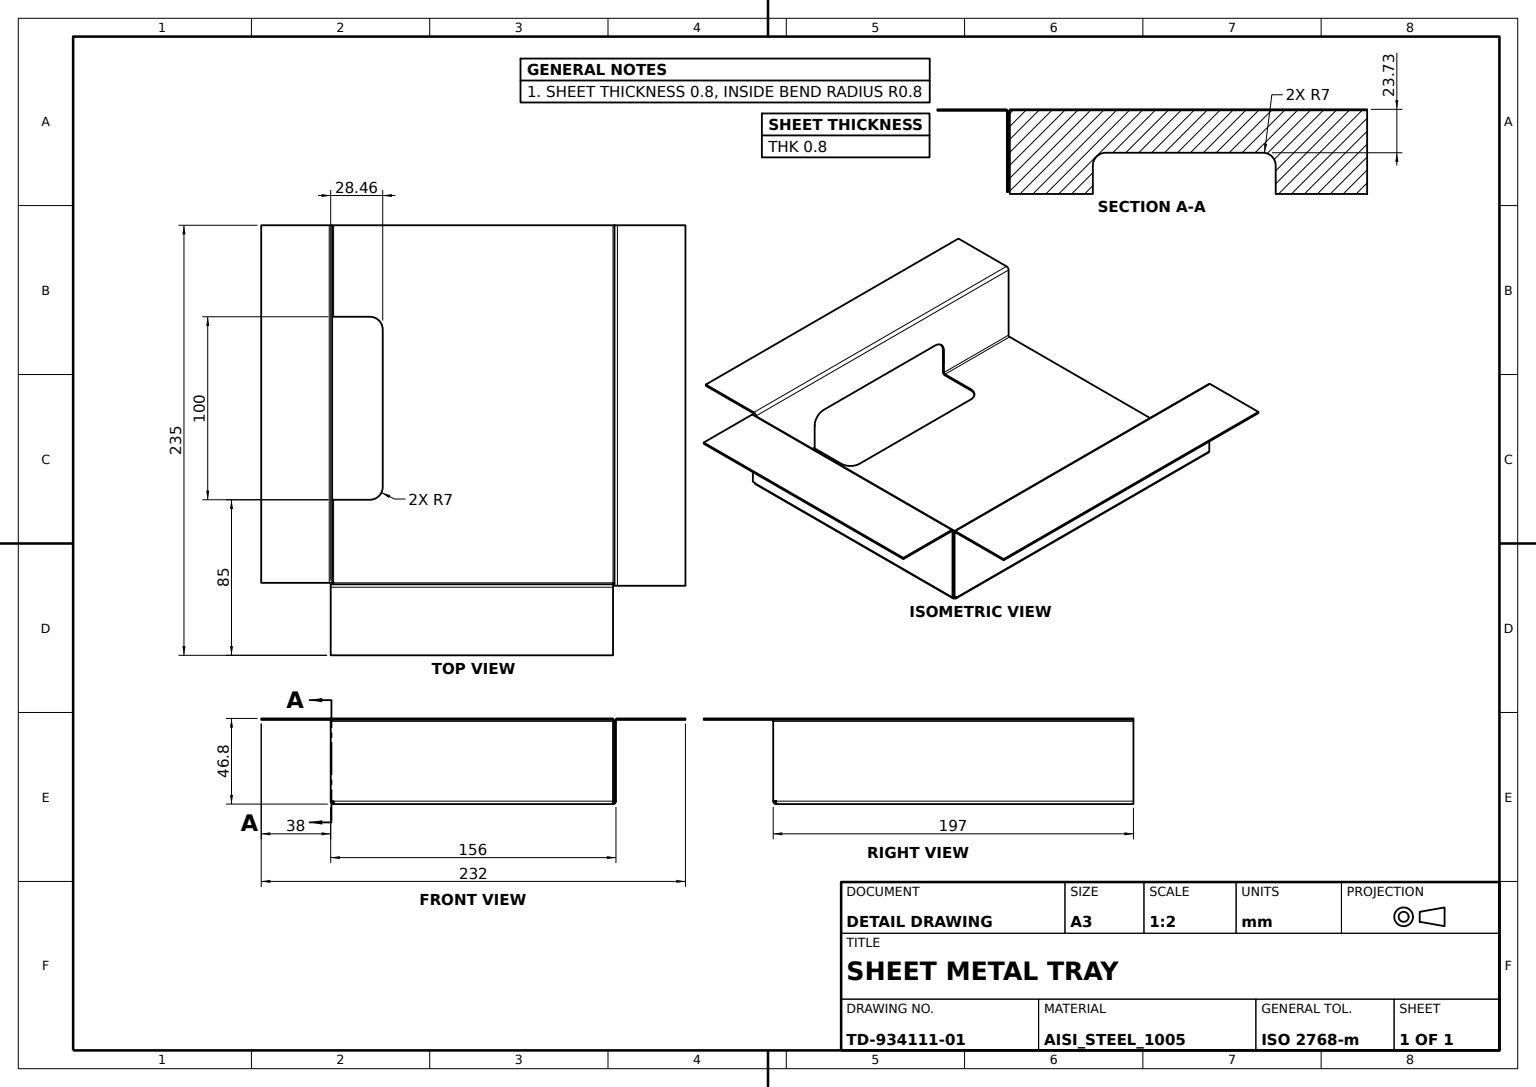
ISO-10303-21;
HEADER;
FILE_DESCRIPTION((''),'2;1');
FILE_NAME('','',(''),(''),'','','');
FILE_SCHEMA(('AUTOMOTIVE_DESIGN'));
ENDSEC;
DATA;
#1=APPLICATION_CONTEXT('');
#2=PRODUCT_CONTEXT('',#1,'mechanical');
#3=PRODUCT('','','',(#2));
#4=PRODUCT_DEFINITION_FORMATION('','',#3);
#5=PRODUCT_DEFINITION_CONTEXT('',#1,'design');
#6=PRODUCT_DEFINITION('','',#4,#5);
#7=PRODUCT_DEFINITION_SHAPE('','',#6);
#8=(LENGTH_UNIT()NAMED_UNIT(*)SI_UNIT(.MILLI.,.METRE.));
#9=(NAMED_UNIT(*)PLANE_ANGLE_UNIT()SI_UNIT($,.RADIAN.));
#10=(NAMED_UNIT(*)SI_UNIT($,.STERADIAN.)SOLID_ANGLE_UNIT());
#11=UNCERTAINTY_MEASURE_WITH_UNIT(LENGTH_MEASURE(0.005),#8,'distance_accuracy_value','');
#12=(GEOMETRIC_REPRESENTATION_CONTEXT(3)GLOBAL_UNCERTAINTY_ASSIGNED_CONTEXT((#11))GLOBAL_UNIT_ASSIGNED_CONTEXT((#8,#9,#10))REPRESENTATION_CONTEXT('',''));
#13=CARTESIAN_POINT('',(77.2,-98.5,1.6));
#14=VERTEX_POINT('',#13);
#15=CARTESIAN_POINT('',(77.2,-98.5,45.2));
#16=VERTEX_POINT('',#15);
#17=DIRECTION('',(0.,0.,1.));
#18=VECTOR('',#17,1000.);
#19=LINE('',#13,#18);
#20=EDGE_CURVE('',#14,#16,#19,.T.);
#21=ORIENTED_EDGE('',*,*,#20,.T.);
#22=CARTESIAN_POINT('',(77.2,98.5,45.2));
#23=VERTEX_POINT('',#22);
#24=DIRECTION('',(0.,1.,0.));
#25=VECTOR('',#24,1000.);
#26=LINE('',#15,#25);
#27=EDGE_CURVE('',#16,#23,#26,.T.);
#28=ORIENTED_EDGE('',*,*,#27,.T.);
#29=CARTESIAN_POINT('',(77.2,98.5,1.6));
#30=VERTEX_POINT('',#29);
#31=LINE('',#29,#18);
#32=EDGE_CURVE('',#30,#23,#31,.T.);
#33=ORIENTED_EDGE('',*,*,#32,.F.);
#34=CARTESIAN_POINT('',(77.2,-96.9,1.6));
#35=VERTEX_POINT('',#34);
#36=DIRECTION('',(0.,-1.,0.));
#37=VECTOR('',#36,1000.);
#38=LINE('',#29,#37);
#39=EDGE_CURVE('',#35,#30,#38,.F.);
#40=ORIENTED_EDGE('',*,*,#39,.F.);
#41=LINE('',#34,#25);
#42=EDGE_CURVE('',#14,#35,#41,.T.);
#43=ORIENTED_EDGE('',*,*,#42,.F.);
#44=EDGE_LOOP('',(#21,#28,#33,#40,#43));
#45=FACE_BOUND('',#44,.T.);
#46=DIRECTION('',(-1.,0.,0.));
#47=AXIS2_PLACEMENT_3D('',#13,#46,#17);
#48=PLANE('',#47);
#49=ADVANCED_FACE('',(#45),#48,.T.);
#50=CARTESIAN_POINT('',(76.4,-98.5,1.6));
#51=VERTEX_POINT('',#50);
#52=CARTESIAN_POINT('',(76.4,-98.5,45.2));
#53=VERTEX_POINT('',#52);
#54=LINE('',#50,#18);
#55=EDGE_CURVE('',#51,#53,#54,.T.);
#56=ORIENTED_EDGE('',*,*,#55,.F.);
#57=CARTESIAN_POINT('',(76.4,-96.9,0.));
#58=VERTEX_POINT('',#57);
#59=CARTESIAN_POINT('',(76.4,-96.9,1.6));
#60=AXIS2_PLACEMENT_3D('',#59,#46,#17);
#61=CIRCLE('',#60,1.6);
#62=EDGE_CURVE('',#58,#51,#61,.T.);
#63=ORIENTED_EDGE('',*,*,#62,.F.);
#64=CARTESIAN_POINT('',(76.4,-96.9,0.8));
#65=VERTEX_POINT('',#64);
#66=LINE('',#59,#18);
#67=EDGE_CURVE('',#65,#58,#66,.F.);
#68=ORIENTED_EDGE('',*,*,#67,.F.);
#69=CARTESIAN_POINT('',(76.4,-97.7,1.6));
#70=VERTEX_POINT('',#69);
#71=AXIS2_PLACEMENT_3D('',#59,#46,#36);
#72=CIRCLE('',#71,0.8);
#73=EDGE_CURVE('',#65,#70,#72,.T.);
#74=ORIENTED_EDGE('',*,*,#73,.T.);
#75=CARTESIAN_POINT('',(76.4,-97.7,45.2));
#76=VERTEX_POINT('',#75);
#77=LINE('',#69,#18);
#78=EDGE_CURVE('',#70,#76,#77,.T.);
#79=ORIENTED_EDGE('',*,*,#78,.T.);
#80=CARTESIAN_POINT('',(76.4,-99.3,46.8));
#81=VERTEX_POINT('',#80);
#82=CARTESIAN_POINT('',(76.4,-99.3,45.2));
#83=DIRECTION('',(1.,0.,0.));
#84=AXIS2_PLACEMENT_3D('',#82,#83,#36);
#85=CIRCLE('',#84,1.6);
#86=EDGE_CURVE('',#76,#81,#85,.T.);
#87=ORIENTED_EDGE('',*,*,#86,.T.);
#88=CARTESIAN_POINT('',(76.4,-136.5,46.8));
#89=VERTEX_POINT('',#88);
#90=LINE('',#80,#25);
#91=EDGE_CURVE('',#81,#89,#90,.F.);
#92=ORIENTED_EDGE('',*,*,#91,.T.);
#93=CARTESIAN_POINT('',(76.4,-136.5,46.));
#94=VERTEX_POINT('',#93);
#95=DIRECTION('',(0.,0.,-1.));
#96=VECTOR('',#95,1000.);
#97=LINE('',#93,#96);
#98=EDGE_CURVE('',#89,#94,#97,.T.);
#99=ORIENTED_EDGE('',*,*,#98,.T.);
#100=CARTESIAN_POINT('',(76.4,-99.3,46.));
#101=VERTEX_POINT('',#100);
#102=LINE('',#100,#37);
#103=EDGE_CURVE('',#101,#94,#102,.T.);
#104=ORIENTED_EDGE('',*,*,#103,.F.);
#105=AXIS2_PLACEMENT_3D('',#82,#83,#95);
#106=CIRCLE('',#105,0.8);
#107=EDGE_CURVE('',#53,#101,#106,.T.);
#108=ORIENTED_EDGE('',*,*,#107,.F.);
#109=EDGE_LOOP('',(#56,#63,#68,#74,#79,#87,#92,#99,#104,#108));
#110=FACE_BOUND('',#109,.T.);
#111=AXIS2_PLACEMENT_3D('',#59,#83,#24);
#112=PLANE('',#111);
#113=ADVANCED_FACE('',(#110),#112,.T.);
#114=ORIENTED_EDGE('',*,*,#67,.T.);
#115=CARTESIAN_POINT('',(78.,-96.9,1.6));
#116=VERTEX_POINT('',#115);
#117=AXIS2_PLACEMENT_3D('',#59,#24,#17);
#118=CIRCLE('',#117,1.6);
#119=EDGE_CURVE('',#116,#58,#118,.T.);
#120=ORIENTED_EDGE('',*,*,#119,.F.);
#121=VECTOR('',#83,1000.);
#122=LINE('',#115,#121);
#123=EDGE_CURVE('',#116,#35,#122,.F.);
#124=ORIENTED_EDGE('',*,*,#123,.T.);
#125=AXIS2_PLACEMENT_3D('',#59,#36,#83);
#126=CIRCLE('',#125,0.8);
#127=EDGE_CURVE('',#35,#65,#126,.F.);
#128=ORIENTED_EDGE('',*,*,#127,.T.);
#129=EDGE_LOOP('',(#114,#120,#124,#128));
#130=FACE_BOUND('',#129,.T.);
#131=PLANE('',#125);
#132=ADVANCED_FACE('',(#130),#131,.T.);
#133=CARTESIAN_POINT('',(-116.,-96.9,46.));
#134=VERTEX_POINT('',#133);
#135=CARTESIAN_POINT('',(-116.,98.5,46.));
#136=VERTEX_POINT('',#135);
#137=LINE('',#133,#25);
#138=EDGE_CURVE('',#134,#136,#137,.T.);
#139=ORIENTED_EDGE('',*,*,#138,.T.);
#140=CARTESIAN_POINT('',(-78.8,98.5,46.));
#141=VERTEX_POINT('',#140);
#142=VECTOR('',#46,1000.);
#143=LINE('',#140,#142);
#144=EDGE_CURVE('',#141,#136,#143,.T.);
#145=ORIENTED_EDGE('',*,*,#144,.F.);
#146=CARTESIAN_POINT('',(-78.8,-96.9,46.));
#147=VERTEX_POINT('',#146);
#148=LINE('',#146,#25);
#149=EDGE_CURVE('',#147,#141,#148,.T.);
#150=ORIENTED_EDGE('',*,*,#149,.F.);
#151=LINE('',#146,#142);
#152=EDGE_CURVE('',#147,#134,#151,.T.);
#153=ORIENTED_EDGE('',*,*,#152,.T.);
#154=EDGE_LOOP('',(#139,#145,#150,#153));
#155=FACE_BOUND('',#154,.T.);
#156=AXIS2_PLACEMENT_3D('',#146,#95,#46);
#157=PLANE('',#156);
#158=ADVANCED_FACE('',(#155),#157,.T.);
#159=CARTESIAN_POINT('',(-76.4,-51.5,0.));
#160=VERTEX_POINT('',#159);
#161=CARTESIAN_POINT('',(-78.,-51.5,1.6));
#162=VERTEX_POINT('',#161);
#163=CARTESIAN_POINT('',(-76.4,-51.5,1.6));
#164=AXIS2_PLACEMENT_3D('',#163,#24,#17);
#165=CIRCLE('',#164,1.6);
#166=EDGE_CURVE('',#160,#162,#165,.T.);
#167=ORIENTED_EDGE('',*,*,#166,.T.);
#168=CARTESIAN_POINT('',(-78.,-51.5,16.071327));
#169=VERTEX_POINT('',#168);
#170=CARTESIAN_POINT('',(-78.,-51.5,-76.471327));
#171=LINE('',#170,#18);
#172=EDGE_CURVE('',#162,#169,#171,.T.);
#173=ORIENTED_EDGE('',*,*,#172,.T.);
#174=CARTESIAN_POINT('',(-77.2,-51.5,16.071327));
#175=VERTEX_POINT('',#174);
#176=LINE('',#168,#142);
#177=EDGE_CURVE('',#175,#169,#176,.T.);
#178=ORIENTED_EDGE('',*,*,#177,.F.);
#179=CARTESIAN_POINT('',(-77.2,-51.5,1.6));
#180=VERTEX_POINT('',#179);
#181=LINE('',#179,#96);
#182=EDGE_CURVE('',#180,#175,#181,.F.);
#183=ORIENTED_EDGE('',*,*,#182,.F.);
#184=CARTESIAN_POINT('',(-76.4,-51.5,0.8));
#185=VERTEX_POINT('',#184);
#186=AXIS2_PLACEMENT_3D('',#163,#24,#46);
#187=CIRCLE('',#186,0.8);
#188=EDGE_CURVE('',#185,#180,#187,.T.);
#189=ORIENTED_EDGE('',*,*,#188,.F.);
#190=CARTESIAN_POINT('',(-56.542655,-51.5,0.8));
#191=VERTEX_POINT('',#190);
#192=CARTESIAN_POINT('',(-78.071327,-51.5,0.8));
#193=LINE('',#192,#121);
#194=EDGE_CURVE('',#191,#185,#193,.F.);
#195=ORIENTED_EDGE('',*,*,#194,.F.);
#196=CARTESIAN_POINT('',(-56.542655,-51.5,0.));
#197=VERTEX_POINT('',#196);
#198=LINE('',#196,#96);
#199=EDGE_CURVE('',#191,#197,#198,.T.);
#200=ORIENTED_EDGE('',*,*,#199,.T.);
#201=CARTESIAN_POINT('',(0.,-51.5,0.));
#202=LINE('',#201,#142);
#203=EDGE_CURVE('',#197,#160,#202,.T.);
#204=ORIENTED_EDGE('',*,*,#203,.T.);
#205=EDGE_LOOP('',(#167,#173,#178,#183,#189,#195,#200,#204));
#206=FACE_BOUND('',#205,.T.);
#207=CARTESIAN_POINT('',(-78.071327,-51.5,0.));
#208=AXIS2_PLACEMENT_3D('',#207,#24,#46);
#209=PLANE('',#208);
#210=ADVANCED_FACE('',(#206),#209,.T.);
#211=CARTESIAN_POINT('',(-77.2,-96.9,45.2));
#212=VERTEX_POINT('',#211);
#213=CARTESIAN_POINT('',(-78.8,-96.9,46.8));
#214=VERTEX_POINT('',#213);
#215=CARTESIAN_POINT('',(-78.8,-96.9,45.2));
#216=AXIS2_PLACEMENT_3D('',#215,#36,#46);
#217=CIRCLE('',#216,1.6);
#218=EDGE_CURVE('',#212,#214,#217,.T.);
#219=ORIENTED_EDGE('',*,*,#218,.T.);
#220=CARTESIAN_POINT('',(-116.,-96.9,46.8));
#221=VERTEX_POINT('',#220);
#222=LINE('',#213,#142);
#223=EDGE_CURVE('',#214,#221,#222,.T.);
#224=ORIENTED_EDGE('',*,*,#223,.T.);
#225=LINE('',#133,#96);
#226=EDGE_CURVE('',#221,#134,#225,.T.);
#227=ORIENTED_EDGE('',*,*,#226,.T.);
#228=ORIENTED_EDGE('',*,*,#152,.F.);
#229=CARTESIAN_POINT('',(-78.,-96.9,45.2));
#230=VERTEX_POINT('',#229);
#231=AXIS2_PLACEMENT_3D('',#215,#36,#83);
#232=CIRCLE('',#231,0.8);
#233=EDGE_CURVE('',#230,#147,#232,.T.);
#234=ORIENTED_EDGE('',*,*,#233,.F.);
#235=CARTESIAN_POINT('',(-78.,-96.9,1.6));
#236=VERTEX_POINT('',#235);
#237=LINE('',#235,#96);
#238=EDGE_CURVE('',#236,#230,#237,.F.);
#239=ORIENTED_EDGE('',*,*,#238,.F.);
#240=CARTESIAN_POINT('',(-76.4,-96.9,0.));
#241=VERTEX_POINT('',#240);
#242=CARTESIAN_POINT('',(-76.4,-96.9,1.6));
#243=AXIS2_PLACEMENT_3D('',#242,#24,#17);
#244=CIRCLE('',#243,1.6);
#245=EDGE_CURVE('',#241,#236,#244,.T.);
#246=ORIENTED_EDGE('',*,*,#245,.F.);
#247=CARTESIAN_POINT('',(-76.4,-96.9,0.8));
#248=VERTEX_POINT('',#247);
#249=LINE('',#242,#18);
#250=EDGE_CURVE('',#248,#241,#249,.F.);
#251=ORIENTED_EDGE('',*,*,#250,.F.);
#252=CARTESIAN_POINT('',(-77.2,-96.9,1.6));
#253=VERTEX_POINT('',#252);
#254=AXIS2_PLACEMENT_3D('',#242,#24,#46);
#255=CIRCLE('',#254,0.8);
#256=EDGE_CURVE('',#248,#253,#255,.T.);
#257=ORIENTED_EDGE('',*,*,#256,.T.);
#258=LINE('',#252,#18);
#259=EDGE_CURVE('',#253,#212,#258,.T.);
#260=ORIENTED_EDGE('',*,*,#259,.T.);
#261=EDGE_LOOP('',(#219,#224,#227,#228,#234,#239,#246,#251,#257,#260));
#262=FACE_BOUND('',#261,.T.);
#263=ADVANCED_FACE('',(#262),#131,.T.);
#264=CARTESIAN_POINT('',(-78.,-99.3,46.8));
#265=VERTEX_POINT('',#264);
#266=CARTESIAN_POINT('',(-78.,-136.5,46.8));
#267=VERTEX_POINT('',#266);
#268=LINE('',#264,#25);
#269=EDGE_CURVE('',#265,#267,#268,.F.);
#270=ORIENTED_EDGE('',*,*,#269,.F.);
#271=CARTESIAN_POINT('',(-78.,-97.7,45.2));
#272=VERTEX_POINT('',#271);
#273=CARTESIAN_POINT('',(-78.,-99.3,45.2));
#274=AXIS2_PLACEMENT_3D('',#273,#83,#36);
#275=CIRCLE('',#274,1.6);
#276=EDGE_CURVE('',#272,#265,#275,.T.);
#277=ORIENTED_EDGE('',*,*,#276,.F.);
#278=CARTESIAN_POINT('',(-78.,-97.7,1.6));
#279=VERTEX_POINT('',#278);
#280=LINE('',#278,#18);
#281=EDGE_CURVE('',#279,#272,#280,.T.);
#282=ORIENTED_EDGE('',*,*,#281,.F.);
#283=CARTESIAN_POINT('',(-78.,-98.5,1.6));
#284=VERTEX_POINT('',#283);
#285=LINE('',#278,#37);
#286=EDGE_CURVE('',#279,#284,#285,.T.);
#287=ORIENTED_EDGE('',*,*,#286,.T.);
#288=CARTESIAN_POINT('',(-78.,-98.5,45.2));
#289=VERTEX_POINT('',#288);
#290=LINE('',#283,#18);
#291=EDGE_CURVE('',#284,#289,#290,.T.);
#292=ORIENTED_EDGE('',*,*,#291,.T.);
#293=CARTESIAN_POINT('',(-78.,-99.3,46.));
#294=VERTEX_POINT('',#293);
#295=AXIS2_PLACEMENT_3D('',#273,#83,#95);
#296=CIRCLE('',#295,0.8);
#297=EDGE_CURVE('',#289,#294,#296,.T.);
#298=ORIENTED_EDGE('',*,*,#297,.T.);
#299=CARTESIAN_POINT('',(-78.,-136.5,46.));
#300=VERTEX_POINT('',#299);
#301=LINE('',#293,#37);
#302=EDGE_CURVE('',#294,#300,#301,.T.);
#303=ORIENTED_EDGE('',*,*,#302,.T.);
#304=LINE('',#299,#96);
#305=EDGE_CURVE('',#267,#300,#304,.T.);
#306=ORIENTED_EDGE('',*,*,#305,.F.);
#307=EDGE_LOOP('',(#270,#277,#282,#287,#292,#298,#303,#306));
#308=FACE_BOUND('',#307,.T.);
#309=AXIS2_PLACEMENT_3D('',#278,#46,#17);
#310=PLANE('',#309);
#311=ADVANCED_FACE('',(#308),#310,.T.);
#312=CARTESIAN_POINT('',(-49.542655,-44.5,0.8));
#313=VERTEX_POINT('',#312);
#314=CARTESIAN_POINT('',(-56.542655,-44.5,0.8));
#315=AXIS2_PLACEMENT_3D('',#314,#17,#83);
#316=CIRCLE('',#315,7.);
#317=EDGE_CURVE('',#313,#191,#316,.F.);
#318=ORIENTED_EDGE('',*,*,#317,.T.);
#319=ORIENTED_EDGE('',*,*,#194,.T.);
#320=CARTESIAN_POINT('',(-76.4,98.5,0.8));
#321=LINE('',#320,#37);
#322=EDGE_CURVE('',#185,#248,#321,.T.);
#323=ORIENTED_EDGE('',*,*,#322,.T.);
#324=CARTESIAN_POINT('',(-78.,-96.9,0.8));
#325=LINE('',#324,#121);
#326=EDGE_CURVE('',#248,#65,#325,.T.);
#327=ORIENTED_EDGE('',*,*,#326,.T.);
#328=CARTESIAN_POINT('',(76.4,98.5,0.8));
#329=VERTEX_POINT('',#328);
#330=CARTESIAN_POINT('',(76.4,-98.5,0.8));
#331=LINE('',#330,#25);
#332=EDGE_CURVE('',#65,#329,#331,.T.);
#333=ORIENTED_EDGE('',*,*,#332,.T.);
#334=VERTEX_POINT('',#320);
#335=CARTESIAN_POINT('',(78.,98.5,0.8));
#336=LINE('',#335,#142);
#337=EDGE_CURVE('',#329,#334,#336,.T.);
#338=ORIENTED_EDGE('',*,*,#337,.T.);
#339=CARTESIAN_POINT('',(-76.4,48.5,0.8));
#340=VERTEX_POINT('',#339);
#341=EDGE_CURVE('',#334,#340,#321,.T.);
#342=ORIENTED_EDGE('',*,*,#341,.T.);
#343=CARTESIAN_POINT('',(-56.542655,48.5,0.8));
#344=VERTEX_POINT('',#343);
#345=CARTESIAN_POINT('',(-78.071327,48.5,0.8));
#346=LINE('',#345,#121);
#347=EDGE_CURVE('',#340,#344,#346,.T.);
#348=ORIENTED_EDGE('',*,*,#347,.T.);
#349=CARTESIAN_POINT('',(-49.542655,41.5,0.8));
#350=VERTEX_POINT('',#349);
#351=CARTESIAN_POINT('',(-56.542655,41.5,0.8));
#352=AXIS2_PLACEMENT_3D('',#351,#17,#83);
#353=CIRCLE('',#352,7.);
#354=EDGE_CURVE('',#344,#350,#353,.F.);
#355=ORIENTED_EDGE('',*,*,#354,.T.);
#356=CARTESIAN_POINT('',(-49.542655,0.,0.8));
#357=LINE('',#356,#25);
#358=EDGE_CURVE('',#350,#313,#357,.F.);
#359=ORIENTED_EDGE('',*,*,#358,.T.);
#360=EDGE_LOOP('',(#318,#319,#323,#327,#333,#338,#342,#348,#355,#359));
#361=FACE_BOUND('',#360,.T.);
#362=CARTESIAN_POINT('',(0.,0.,0.8));
#363=AXIS2_PLACEMENT_3D('',#362,#17,#83);
#364=PLANE('',#363);
#365=ADVANCED_FACE('',(#361),#364,.T.);
#366=CARTESIAN_POINT('',(-78.,-44.5,23.071327));
#367=VERTEX_POINT('',#366);
#368=CARTESIAN_POINT('',(-78.,41.5,23.071327));
#369=VERTEX_POINT('',#368);
#370=CARTESIAN_POINT('',(-78.,98.5,23.071327));
#371=LINE('',#370,#25);
#372=EDGE_CURVE('',#367,#369,#371,.T.);
#373=ORIENTED_EDGE('',*,*,#372,.T.);
#374=CARTESIAN_POINT('',(-77.2,41.5,23.071327));
#375=VERTEX_POINT('',#374);
#376=LINE('',#368,#142);
#377=EDGE_CURVE('',#375,#369,#376,.T.);
#378=ORIENTED_EDGE('',*,*,#377,.F.);
#379=CARTESIAN_POINT('',(-77.2,-44.5,23.071327));
#380=VERTEX_POINT('',#379);
#381=CARTESIAN_POINT('',(-77.2,98.5,23.071327));
#382=LINE('',#381,#25);
#383=EDGE_CURVE('',#380,#375,#382,.T.);
#384=ORIENTED_EDGE('',*,*,#383,.F.);
#385=LINE('',#366,#142);
#386=EDGE_CURVE('',#380,#367,#385,.T.);
#387=ORIENTED_EDGE('',*,*,#386,.T.);
#388=EDGE_LOOP('',(#373,#378,#384,#387));
#389=FACE_BOUND('',#388,.T.);
#390=AXIS2_PLACEMENT_3D('',#370,#95,#24);
#391=PLANE('',#390);
#392=ADVANCED_FACE('',(#389),#391,.T.);
#393=CARTESIAN_POINT('',(78.8,-98.5,46.8));
#394=VERTEX_POINT('',#393);
#395=CARTESIAN_POINT('',(78.8,-98.5,45.2));
#396=AXIS2_PLACEMENT_3D('',#395,#24,#83);
#397=CIRCLE('',#396,1.6);
#398=EDGE_CURVE('',#16,#394,#397,.T.);
#399=ORIENTED_EDGE('',*,*,#398,.T.);
#400=CARTESIAN_POINT('',(78.8,98.5,46.8));
#401=VERTEX_POINT('',#400);
#402=LINE('',#400,#37);
#403=EDGE_CURVE('',#401,#394,#402,.T.);
#404=ORIENTED_EDGE('',*,*,#403,.F.);
#405=CARTESIAN_POINT('',(78.8,98.5,45.2));
#406=AXIS2_PLACEMENT_3D('',#405,#24,#83);
#407=CIRCLE('',#406,1.6);
#408=EDGE_CURVE('',#23,#401,#407,.T.);
#409=ORIENTED_EDGE('',*,*,#408,.F.);
#410=ORIENTED_EDGE('',*,*,#27,.F.);
#411=EDGE_LOOP('',(#399,#404,#409,#410));
#412=FACE_BOUND('',#411,.T.);
#413=CYLINDRICAL_SURFACE('',#396,1.6);
#414=ADVANCED_FACE('',(#412),#413,.T.);
#415=CARTESIAN_POINT('',(-78.,-96.9,0.));
#416=LINE('',#415,#121);
#417=EDGE_CURVE('',#241,#58,#416,.T.);
#418=ORIENTED_EDGE('',*,*,#417,.F.);
#419=CARTESIAN_POINT('',(-76.4,98.5,0.));
#420=LINE('',#419,#37);
#421=EDGE_CURVE('',#160,#241,#420,.T.);
#422=ORIENTED_EDGE('',*,*,#421,.F.);
#423=ORIENTED_EDGE('',*,*,#203,.F.);
#424=CARTESIAN_POINT('',(-49.542655,-44.5,0.));
#425=VERTEX_POINT('',#424);
#426=CARTESIAN_POINT('',(-56.542655,-44.5,0.));
#427=AXIS2_PLACEMENT_3D('',#426,#17,#83);
#428=CIRCLE('',#427,7.);
#429=EDGE_CURVE('',#425,#197,#428,.F.);
#430=ORIENTED_EDGE('',*,*,#429,.F.);
#431=CARTESIAN_POINT('',(-49.542655,41.5,0.));
#432=VERTEX_POINT('',#431);
#433=CARTESIAN_POINT('',(-49.542655,0.,0.));
#434=LINE('',#433,#37);
#435=EDGE_CURVE('',#432,#425,#434,.T.);
#436=ORIENTED_EDGE('',*,*,#435,.F.);
#437=CARTESIAN_POINT('',(-56.542655,48.5,0.));
#438=VERTEX_POINT('',#437);
#439=CARTESIAN_POINT('',(-56.542655,41.5,0.));
#440=AXIS2_PLACEMENT_3D('',#439,#17,#83);
#441=CIRCLE('',#440,7.);
#442=EDGE_CURVE('',#438,#432,#441,.F.);
#443=ORIENTED_EDGE('',*,*,#442,.F.);
#444=CARTESIAN_POINT('',(-76.4,48.5,0.));
#445=VERTEX_POINT('',#444);
#446=CARTESIAN_POINT('',(0.,48.5,0.));
#447=LINE('',#446,#121);
#448=EDGE_CURVE('',#445,#438,#447,.T.);
#449=ORIENTED_EDGE('',*,*,#448,.F.);
#450=VERTEX_POINT('',#419);
#451=EDGE_CURVE('',#450,#445,#420,.T.);
#452=ORIENTED_EDGE('',*,*,#451,.F.);
#453=CARTESIAN_POINT('',(76.4,98.5,0.));
#454=VERTEX_POINT('',#453);
#455=CARTESIAN_POINT('',(78.,98.5,0.));
#456=LINE('',#455,#142);
#457=EDGE_CURVE('',#454,#450,#456,.T.);
#458=ORIENTED_EDGE('',*,*,#457,.F.);
#459=CARTESIAN_POINT('',(76.4,-98.5,0.));
#460=LINE('',#459,#25);
#461=EDGE_CURVE('',#58,#454,#460,.T.);
#462=ORIENTED_EDGE('',*,*,#461,.F.);
#463=EDGE_LOOP('',(#418,#422,#423,#430,#436,#443,#449,#452,#458,#462));
#464=FACE_BOUND('',#463,.T.);
#465=CARTESIAN_POINT('',(0.,0.,0.));
#466=AXIS2_PLACEMENT_3D('',#465,#17,#83);
#467=PLANE('',#466);
#468=ADVANCED_FACE('',(#464),#467,.F.);
#469=ORIENTED_EDGE('',*,*,#302,.F.);
#470=LINE('',#100,#142);
#471=EDGE_CURVE('',#101,#294,#470,.T.);
#472=ORIENTED_EDGE('',*,*,#471,.F.);
#473=ORIENTED_EDGE('',*,*,#103,.T.);
#474=LINE('',#93,#142);
#475=EDGE_CURVE('',#94,#300,#474,.T.);
#476=ORIENTED_EDGE('',*,*,#475,.T.);
#477=EDGE_LOOP('',(#469,#472,#473,#476));
#478=FACE_BOUND('',#477,.T.);
#479=AXIS2_PLACEMENT_3D('',#100,#95,#24);
#480=PLANE('',#479);
#481=ADVANCED_FACE('',(#478),#480,.T.);
#482=CARTESIAN_POINT('',(116.,98.5,46.8));
#483=VERTEX_POINT('',#482);
#484=CARTESIAN_POINT('',(116.,-98.5,46.8));
#485=VERTEX_POINT('',#484);
#486=LINE('',#482,#25);
#487=EDGE_CURVE('',#483,#485,#486,.F.);
#488=ORIENTED_EDGE('',*,*,#487,.F.);
#489=LINE('',#400,#142);
#490=EDGE_CURVE('',#401,#483,#489,.F.);
#491=ORIENTED_EDGE('',*,*,#490,.F.);
#492=ORIENTED_EDGE('',*,*,#403,.T.);
#493=LINE('',#393,#142);
#494=EDGE_CURVE('',#394,#485,#493,.F.);
#495=ORIENTED_EDGE('',*,*,#494,.T.);
#496=EDGE_LOOP('',(#488,#491,#492,#495));
#497=FACE_BOUND('',#496,.T.);
#498=AXIS2_PLACEMENT_3D('',#400,#95,#46);
#499=PLANE('',#498);
#500=ADVANCED_FACE('',(#497),#499,.F.);
#501=ORIENTED_EDGE('',*,*,#358,.F.);
#502=LINE('',#431,#96);
#503=EDGE_CURVE('',#350,#432,#502,.T.);
#504=ORIENTED_EDGE('',*,*,#503,.T.);
#505=ORIENTED_EDGE('',*,*,#435,.T.);
#506=LINE('',#424,#96);
#507=EDGE_CURVE('',#313,#425,#506,.T.);
#508=ORIENTED_EDGE('',*,*,#507,.F.);
#509=EDGE_LOOP('',(#501,#504,#505,#508));
#510=FACE_BOUND('',#509,.T.);
#511=AXIS2_PLACEMENT_3D('',#433,#46,#36);
#512=PLANE('',#511);
#513=ADVANCED_FACE('',(#510),#512,.T.);
#514=CARTESIAN_POINT('',(116.,-98.5,46.));
#515=VERTEX_POINT('',#514);
#516=LINE('',#514,#96);
#517=EDGE_CURVE('',#485,#515,#516,.T.);
#518=ORIENTED_EDGE('',*,*,#517,.T.);
#519=CARTESIAN_POINT('',(116.,98.5,46.));
#520=VERTEX_POINT('',#519);
#521=LINE('',#519,#37);
#522=EDGE_CURVE('',#520,#515,#521,.T.);
#523=ORIENTED_EDGE('',*,*,#522,.F.);
#524=LINE('',#519,#96);
#525=EDGE_CURVE('',#483,#520,#524,.T.);
#526=ORIENTED_EDGE('',*,*,#525,.F.);
#527=ORIENTED_EDGE('',*,*,#487,.T.);
#528=EDGE_LOOP('',(#518,#523,#526,#527));
#529=FACE_BOUND('',#528,.T.);
#530=AXIS2_PLACEMENT_3D('',#519,#83,#36);
#531=PLANE('',#530);
#532=ADVANCED_FACE('',(#529),#531,.T.);
#533=ORIENTED_EDGE('',*,*,#322,.F.);
#534=ORIENTED_EDGE('',*,*,#188,.T.);
#535=CARTESIAN_POINT('',(-77.2,98.5,1.6));
#536=LINE('',#535,#37);
#537=EDGE_CURVE('',#180,#253,#536,.T.);
#538=ORIENTED_EDGE('',*,*,#537,.T.);
#539=ORIENTED_EDGE('',*,*,#256,.F.);
#540=EDGE_LOOP('',(#533,#534,#538,#539));
#541=FACE_BOUND('',#540,.T.);
#542=CYLINDRICAL_SURFACE('',#243,0.8);
#543=ADVANCED_FACE('',(#541),#542,.F.);
#544=CARTESIAN_POINT('',(-76.4,-98.5,1.6));
#545=VERTEX_POINT('',#544);
#546=AXIS2_PLACEMENT_3D('',#242,#83,#17);
#547=CIRCLE('',#546,1.6);
#548=EDGE_CURVE('',#545,#241,#547,.T.);
#549=ORIENTED_EDGE('',*,*,#548,.F.);
#550=CARTESIAN_POINT('',(-76.4,-97.7,1.6));
#551=VERTEX_POINT('',#550);
#552=LINE('',#544,#37);
#553=EDGE_CURVE('',#545,#551,#552,.F.);
#554=ORIENTED_EDGE('',*,*,#553,.T.);
#555=AXIS2_PLACEMENT_3D('',#242,#46,#36);
#556=CIRCLE('',#555,0.8);
#557=EDGE_CURVE('',#551,#248,#556,.F.);
#558=ORIENTED_EDGE('',*,*,#557,.T.);
#559=ORIENTED_EDGE('',*,*,#250,.T.);
#560=EDGE_LOOP('',(#549,#554,#558,#559));
#561=FACE_BOUND('',#560,.T.);
#562=PLANE('',#555);
#563=ADVANCED_FACE('',(#561),#562,.T.);
#564=CARTESIAN_POINT('',(78.8,-98.5,46.));
#565=VERTEX_POINT('',#564);
#566=LINE('',#564,#121);
#567=EDGE_CURVE('',#565,#515,#566,.T.);
#568=ORIENTED_EDGE('',*,*,#567,.F.);
#569=CARTESIAN_POINT('',(78.8,98.5,46.));
#570=VERTEX_POINT('',#569);
#571=LINE('',#569,#37);
#572=EDGE_CURVE('',#570,#565,#571,.T.);
#573=ORIENTED_EDGE('',*,*,#572,.F.);
#574=LINE('',#569,#121);
#575=EDGE_CURVE('',#570,#520,#574,.T.);
#576=ORIENTED_EDGE('',*,*,#575,.T.);
#577=ORIENTED_EDGE('',*,*,#522,.T.);
#578=EDGE_LOOP('',(#568,#573,#576,#577));
#579=FACE_BOUND('',#578,.T.);
#580=AXIS2_PLACEMENT_3D('',#569,#95,#46);
#581=PLANE('',#580);
#582=ADVANCED_FACE('',(#579),#581,.T.);
#583=ORIENTED_EDGE('',*,*,#297,.F.);
#584=LINE('',#288,#121);
#585=EDGE_CURVE('',#289,#53,#584,.T.);
#586=ORIENTED_EDGE('',*,*,#585,.T.);
#587=ORIENTED_EDGE('',*,*,#107,.T.);
#588=ORIENTED_EDGE('',*,*,#471,.T.);
#589=EDGE_LOOP('',(#583,#586,#587,#588));
#590=FACE_BOUND('',#589,.T.);
#591=CYLINDRICAL_SURFACE('',#274,0.8);
#592=ADVANCED_FACE('',(#590),#591,.F.);
#593=ORIENTED_EDGE('',*,*,#386,.F.);
#594=CARTESIAN_POINT('',(-77.2,-44.5,16.071327));
#595=AXIS2_PLACEMENT_3D('',#594,#83,#95);
#596=CIRCLE('',#595,7.);
#597=EDGE_CURVE('',#175,#380,#596,.F.);
#598=ORIENTED_EDGE('',*,*,#597,.F.);
#599=ORIENTED_EDGE('',*,*,#177,.T.);
#600=CARTESIAN_POINT('',(-78.,-44.5,16.071327));
#601=AXIS2_PLACEMENT_3D('',#600,#83,#95);
#602=CIRCLE('',#601,7.);
#603=EDGE_CURVE('',#169,#367,#602,.F.);
#604=ORIENTED_EDGE('',*,*,#603,.T.);
#605=EDGE_LOOP('',(#593,#598,#599,#604));
#606=FACE_BOUND('',#605,.T.);
#607=CYLINDRICAL_SURFACE('',#601,7.);
#608=ADVANCED_FACE('',(#606),#607,.F.);
#609=CARTESIAN_POINT('',(78.,98.5,1.6));
#610=VERTEX_POINT('',#609);
#611=LINE('',#115,#25);
#612=EDGE_CURVE('',#116,#610,#611,.T.);
#613=ORIENTED_EDGE('',*,*,#612,.F.);
#614=ORIENTED_EDGE('',*,*,#119,.T.);
#615=ORIENTED_EDGE('',*,*,#461,.T.);
#616=CARTESIAN_POINT('',(76.4,98.5,1.6));
#617=AXIS2_PLACEMENT_3D('',#616,#36,#17);
#618=CIRCLE('',#617,1.6);
#619=EDGE_CURVE('',#454,#610,#618,.T.);
#620=ORIENTED_EDGE('',*,*,#619,.T.);
#621=EDGE_LOOP('',(#613,#614,#615,#620));
#622=FACE_BOUND('',#621,.T.);
#623=CYLINDRICAL_SURFACE('',#617,1.6);
#624=ADVANCED_FACE('',(#622),#623,.T.);
#625=ORIENTED_EDGE('',*,*,#281,.T.);
#626=LINE('',#271,#121);
#627=EDGE_CURVE('',#272,#76,#626,.T.);
#628=ORIENTED_EDGE('',*,*,#627,.T.);
#629=ORIENTED_EDGE('',*,*,#78,.F.);
#630=LINE('',#69,#142);
#631=EDGE_CURVE('',#551,#70,#630,.F.);
#632=ORIENTED_EDGE('',*,*,#631,.F.);
#633=LINE('',#550,#121);
#634=EDGE_CURVE('',#279,#551,#633,.T.);
#635=ORIENTED_EDGE('',*,*,#634,.F.);
#636=EDGE_LOOP('',(#625,#628,#629,#632,#635));
#637=FACE_BOUND('',#636,.T.);
#638=AXIS2_PLACEMENT_3D('',#278,#24,#17);
#639=PLANE('',#638);
#640=ADVANCED_FACE('',(#637),#639,.T.);
#641=ORIENTED_EDGE('',*,*,#226,.F.);
#642=CARTESIAN_POINT('',(-116.,98.5,46.8));
#643=VERTEX_POINT('',#642);
#644=LINE('',#220,#25);
#645=EDGE_CURVE('',#221,#643,#644,.T.);
#646=ORIENTED_EDGE('',*,*,#645,.T.);
#647=LINE('',#135,#96);
#648=EDGE_CURVE('',#643,#136,#647,.T.);
#649=ORIENTED_EDGE('',*,*,#648,.T.);
#650=ORIENTED_EDGE('',*,*,#138,.F.);
#651=EDGE_LOOP('',(#641,#646,#649,#650));
#652=FACE_BOUND('',#651,.T.);
#653=AXIS2_PLACEMENT_3D('',#133,#46,#24);
#654=PLANE('',#653);
#655=ADVANCED_FACE('',(#652),#654,.T.);
#656=CARTESIAN_POINT('',(-78.8,98.5,46.8));
#657=VERTEX_POINT('',#656);
#658=LINE('',#656,#142);
#659=EDGE_CURVE('',#657,#643,#658,.T.);
#660=ORIENTED_EDGE('',*,*,#659,.T.);
#661=ORIENTED_EDGE('',*,*,#645,.F.);
#662=ORIENTED_EDGE('',*,*,#223,.F.);
#663=LINE('',#213,#25);
#664=EDGE_CURVE('',#214,#657,#663,.T.);
#665=ORIENTED_EDGE('',*,*,#664,.T.);
#666=EDGE_LOOP('',(#660,#661,#662,#665));
#667=FACE_BOUND('',#666,.T.);
#668=AXIS2_PLACEMENT_3D('',#213,#95,#46);
#669=PLANE('',#668);
#670=ADVANCED_FACE('',(#667),#669,.F.);
#671=LINE('',#544,#121);
#672=EDGE_CURVE('',#545,#51,#671,.T.);
#673=ORIENTED_EDGE('',*,*,#672,.T.);
#674=ORIENTED_EDGE('',*,*,#55,.T.);
#675=ORIENTED_EDGE('',*,*,#585,.F.);
#676=ORIENTED_EDGE('',*,*,#291,.F.);
#677=LINE('',#283,#121);
#678=EDGE_CURVE('',#284,#545,#677,.T.);
#679=ORIENTED_EDGE('',*,*,#678,.T.);
#680=EDGE_LOOP('',(#673,#674,#675,#676,#679));
#681=FACE_BOUND('',#680,.T.);
#682=AXIS2_PLACEMENT_3D('',#283,#24,#17);
#683=PLANE('',#682);
#684=ADVANCED_FACE('',(#681),#683,.F.);
#685=LINE('',#437,#96);
#686=EDGE_CURVE('',#344,#438,#685,.T.);
#687=ORIENTED_EDGE('',*,*,#686,.T.);
#688=ORIENTED_EDGE('',*,*,#442,.T.);
#689=ORIENTED_EDGE('',*,*,#503,.F.);
#690=ORIENTED_EDGE('',*,*,#354,.F.);
#691=EDGE_LOOP('',(#687,#688,#689,#690));
#692=FACE_BOUND('',#691,.T.);
#693=CYLINDRICAL_SURFACE('',#440,7.);
#694=ADVANCED_FACE('',(#692),#693,.F.);
#695=LINE('',#88,#121);
#696=EDGE_CURVE('',#89,#267,#695,.F.);
#697=ORIENTED_EDGE('',*,*,#696,.F.);
#698=ORIENTED_EDGE('',*,*,#91,.F.);
#699=LINE('',#80,#142);
#700=EDGE_CURVE('',#81,#265,#699,.T.);
#701=ORIENTED_EDGE('',*,*,#700,.T.);
#702=ORIENTED_EDGE('',*,*,#269,.T.);
#703=EDGE_LOOP('',(#697,#698,#701,#702));
#704=FACE_BOUND('',#703,.T.);
#705=AXIS2_PLACEMENT_3D('',#80,#95,#24);
#706=PLANE('',#705);
#707=ADVANCED_FACE('',(#704),#706,.F.);
#708=CARTESIAN_POINT('',(-77.2,98.5,45.2));
#709=VERTEX_POINT('',#708);
#710=CARTESIAN_POINT('',(-78.8,98.5,45.2));
#711=AXIS2_PLACEMENT_3D('',#710,#36,#46);
#712=CIRCLE('',#711,1.6);
#713=EDGE_CURVE('',#709,#657,#712,.T.);
#714=ORIENTED_EDGE('',*,*,#713,.T.);
#715=ORIENTED_EDGE('',*,*,#664,.F.);
#716=ORIENTED_EDGE('',*,*,#218,.F.);
#717=LINE('',#708,#37);
#718=EDGE_CURVE('',#709,#212,#717,.T.);
#719=ORIENTED_EDGE('',*,*,#718,.F.);
#720=EDGE_LOOP('',(#714,#715,#716,#719));
#721=FACE_BOUND('',#720,.T.);
#722=CYLINDRICAL_SURFACE('',#711,1.6);
#723=ADVANCED_FACE('',(#721),#722,.T.);
#724=CARTESIAN_POINT('',(-78.,48.5,1.6));
#725=VERTEX_POINT('',#724);
#726=CARTESIAN_POINT('',(-76.4,48.5,1.6));
#727=AXIS2_PLACEMENT_3D('',#726,#36,#17);
#728=CIRCLE('',#727,1.6);
#729=EDGE_CURVE('',#725,#445,#728,.T.);
#730=ORIENTED_EDGE('',*,*,#729,.F.);
#731=CARTESIAN_POINT('',(-78.,98.5,1.6));
#732=VERTEX_POINT('',#731);
#733=LINE('',#731,#37);
#734=EDGE_CURVE('',#732,#725,#733,.T.);
#735=ORIENTED_EDGE('',*,*,#734,.F.);
#736=CARTESIAN_POINT('',(-76.4,98.5,1.6));
#737=AXIS2_PLACEMENT_3D('',#736,#24,#17);
#738=CIRCLE('',#737,1.6);
#739=EDGE_CURVE('',#450,#732,#738,.T.);
#740=ORIENTED_EDGE('',*,*,#739,.F.);
#741=ORIENTED_EDGE('',*,*,#451,.T.);
#742=EDGE_LOOP('',(#730,#735,#740,#741));
#743=FACE_BOUND('',#742,.T.);
#744=CYLINDRICAL_SURFACE('',#243,1.6);
#745=ADVANCED_FACE('',(#743),#744,.T.);
#746=ORIENTED_EDGE('',*,*,#259,.F.);
#747=ORIENTED_EDGE('',*,*,#537,.F.);
#748=ORIENTED_EDGE('',*,*,#182,.T.);
#749=ORIENTED_EDGE('',*,*,#597,.T.);
#750=ORIENTED_EDGE('',*,*,#383,.T.);
#751=CARTESIAN_POINT('',(-77.2,48.5,16.071327));
#752=VERTEX_POINT('',#751);
#753=CARTESIAN_POINT('',(-77.2,41.5,16.071327));
#754=AXIS2_PLACEMENT_3D('',#753,#83,#95);
#755=CIRCLE('',#754,7.);
#756=EDGE_CURVE('',#375,#752,#755,.F.);
#757=ORIENTED_EDGE('',*,*,#756,.T.);
#758=CARTESIAN_POINT('',(-77.2,48.5,1.6));
#759=VERTEX_POINT('',#758);
#760=LINE('',#758,#96);
#761=EDGE_CURVE('',#752,#759,#760,.T.);
#762=ORIENTED_EDGE('',*,*,#761,.T.);
#763=VERTEX_POINT('',#535);
#764=EDGE_CURVE('',#763,#759,#536,.T.);
#765=ORIENTED_EDGE('',*,*,#764,.F.);
#766=LINE('',#535,#18);
#767=EDGE_CURVE('',#763,#709,#766,.T.);
#768=ORIENTED_EDGE('',*,*,#767,.T.);
#769=ORIENTED_EDGE('',*,*,#718,.T.);
#770=EDGE_LOOP('',(#746,#747,#748,#749,#750,#757,#762,#765,#768,#769));
#771=FACE_BOUND('',#770,.T.);
#772=AXIS2_PLACEMENT_3D('',#535,#83,#95);
#773=PLANE('',#772);
#774=ADVANCED_FACE('',(#771),#773,.T.);
#775=ORIENTED_EDGE('',*,*,#421,.T.);
#776=ORIENTED_EDGE('',*,*,#245,.T.);
#777=EDGE_CURVE('',#162,#236,#733,.T.);
#778=ORIENTED_EDGE('',*,*,#777,.F.);
#779=ORIENTED_EDGE('',*,*,#166,.F.);
#780=EDGE_LOOP('',(#775,#776,#778,#779));
#781=FACE_BOUND('',#780,.T.);
#782=ADVANCED_FACE('',(#781),#744,.T.);
#783=ORIENTED_EDGE('',*,*,#123,.F.);
#784=CARTESIAN_POINT('',(78.,-98.5,1.6));
#785=VERTEX_POINT('',#784);
#786=LINE('',#784,#25);
#787=EDGE_CURVE('',#785,#116,#786,.T.);
#788=ORIENTED_EDGE('',*,*,#787,.F.);
#789=LINE('',#283,#142);
#790=EDGE_CURVE('',#785,#14,#789,.T.);
#791=ORIENTED_EDGE('',*,*,#790,.T.);
#792=ORIENTED_EDGE('',*,*,#42,.T.);
#793=EDGE_LOOP('',(#783,#788,#791,#792));
#794=FACE_BOUND('',#793,.T.);
#795=CARTESIAN_POINT('',(0.,0.,1.6));
#796=AXIS2_PLACEMENT_3D('',#795,#95,#24);
#797=PLANE('',#796);
#798=ADVANCED_FACE('',(#794),#797,.T.);
#799=ORIENTED_EDGE('',*,*,#787,.T.);
#800=ORIENTED_EDGE('',*,*,#612,.T.);
#801=CARTESIAN_POINT('',(78.,98.5,45.2));
#802=VERTEX_POINT('',#801);
#803=LINE('',#609,#18);
#804=EDGE_CURVE('',#610,#802,#803,.T.);
#805=ORIENTED_EDGE('',*,*,#804,.T.);
#806=CARTESIAN_POINT('',(78.,-98.5,45.2));
#807=VERTEX_POINT('',#806);
#808=LINE('',#806,#25);
#809=EDGE_CURVE('',#807,#802,#808,.T.);
#810=ORIENTED_EDGE('',*,*,#809,.F.);
#811=LINE('',#784,#18);
#812=EDGE_CURVE('',#785,#807,#811,.T.);
#813=ORIENTED_EDGE('',*,*,#812,.F.);
#814=EDGE_LOOP('',(#799,#800,#805,#810,#813));
#815=FACE_BOUND('',#814,.T.);
#816=AXIS2_PLACEMENT_3D('',#784,#46,#17);
#817=PLANE('',#816);
#818=ADVANCED_FACE('',(#815),#817,.F.);
#819=ORIENTED_EDGE('',*,*,#233,.T.);
#820=ORIENTED_EDGE('',*,*,#149,.T.);
#821=CARTESIAN_POINT('',(-78.,98.5,45.2));
#822=VERTEX_POINT('',#821);
#823=AXIS2_PLACEMENT_3D('',#710,#36,#83);
#824=CIRCLE('',#823,0.8);
#825=EDGE_CURVE('',#822,#141,#824,.T.);
#826=ORIENTED_EDGE('',*,*,#825,.F.);
#827=LINE('',#821,#37);
#828=EDGE_CURVE('',#822,#230,#827,.T.);
#829=ORIENTED_EDGE('',*,*,#828,.T.);
#830=EDGE_LOOP('',(#819,#820,#826,#829));
#831=FACE_BOUND('',#830,.T.);
#832=CYLINDRICAL_SURFACE('',#711,0.8);
#833=ADVANCED_FACE('',(#831),#832,.F.);
#834=ORIENTED_EDGE('',*,*,#627,.F.);
#835=ORIENTED_EDGE('',*,*,#276,.T.);
#836=ORIENTED_EDGE('',*,*,#700,.F.);
#837=ORIENTED_EDGE('',*,*,#86,.F.);
#838=EDGE_LOOP('',(#834,#835,#836,#837));
#839=FACE_BOUND('',#838,.T.);
#840=CYLINDRICAL_SURFACE('',#274,1.6);
#841=ADVANCED_FACE('',(#839),#840,.T.);
#842=ORIENTED_EDGE('',*,*,#98,.F.);
#843=ORIENTED_EDGE('',*,*,#696,.T.);
#844=ORIENTED_EDGE('',*,*,#305,.T.);
#845=ORIENTED_EDGE('',*,*,#475,.F.);
#846=EDGE_LOOP('',(#842,#843,#844,#845));
#847=FACE_BOUND('',#846,.T.);
#848=AXIS2_PLACEMENT_3D('',#93,#36,#46);
#849=PLANE('',#848);
#850=ADVANCED_FACE('',(#847),#849,.T.);
#851=ORIENTED_EDGE('',*,*,#62,.T.);
#852=ORIENTED_EDGE('',*,*,#672,.F.);
#853=ORIENTED_EDGE('',*,*,#548,.T.);
#854=ORIENTED_EDGE('',*,*,#417,.T.);
#855=EDGE_LOOP('',(#851,#852,#853,#854));
#856=FACE_BOUND('',#855,.T.);
#857=CYLINDRICAL_SURFACE('',#60,1.6);
#858=ADVANCED_FACE('',(#856),#857,.T.);
#859=ORIENTED_EDGE('',*,*,#429,.T.);
#860=ORIENTED_EDGE('',*,*,#199,.F.);
#861=ORIENTED_EDGE('',*,*,#317,.F.);
#862=ORIENTED_EDGE('',*,*,#507,.T.);
#863=EDGE_LOOP('',(#859,#860,#861,#862));
#864=FACE_BOUND('',#863,.T.);
#865=CYLINDRICAL_SURFACE('',#427,7.);
#866=ADVANCED_FACE('',(#864),#865,.F.);
#867=ORIENTED_EDGE('',*,*,#812,.T.);
#868=AXIS2_PLACEMENT_3D('',#395,#24,#46);
#869=CIRCLE('',#868,0.8);
#870=EDGE_CURVE('',#807,#565,#869,.T.);
#871=ORIENTED_EDGE('',*,*,#870,.T.);
#872=ORIENTED_EDGE('',*,*,#567,.T.);
#873=ORIENTED_EDGE('',*,*,#517,.F.);
#874=ORIENTED_EDGE('',*,*,#494,.F.);
#875=ORIENTED_EDGE('',*,*,#398,.F.);
#876=ORIENTED_EDGE('',*,*,#20,.F.);
#877=ORIENTED_EDGE('',*,*,#790,.F.);
#878=EDGE_LOOP('',(#867,#871,#872,#873,#874,#875,#876,#877));
#879=FACE_BOUND('',#878,.T.);
#880=CARTESIAN_POINT('',(-78.,-98.5,0.8));
#881=AXIS2_PLACEMENT_3D('',#880,#24,#17);
#882=PLANE('',#881);
#883=ADVANCED_FACE('',(#879),#882,.F.);
#884=ORIENTED_EDGE('',*,*,#377,.T.);
#885=CARTESIAN_POINT('',(-78.,48.5,16.071327));
#886=VERTEX_POINT('',#885);
#887=CARTESIAN_POINT('',(-78.,41.5,16.071327));
#888=AXIS2_PLACEMENT_3D('',#887,#83,#95);
#889=CIRCLE('',#888,7.);
#890=EDGE_CURVE('',#369,#886,#889,.F.);
#891=ORIENTED_EDGE('',*,*,#890,.T.);
#892=LINE('',#885,#142);
#893=EDGE_CURVE('',#752,#886,#892,.T.);
#894=ORIENTED_EDGE('',*,*,#893,.F.);
#895=ORIENTED_EDGE('',*,*,#756,.F.);
#896=EDGE_LOOP('',(#884,#891,#894,#895));
#897=FACE_BOUND('',#896,.T.);
#898=CYLINDRICAL_SURFACE('',#888,7.);
#899=ADVANCED_FACE('',(#897),#898,.F.);
#900=CARTESIAN_POINT('',(-78.,48.5,-76.471327));
#901=LINE('',#900,#96);
#902=EDGE_CURVE('',#886,#725,#901,.T.);
#903=ORIENTED_EDGE('',*,*,#902,.T.);
#904=ORIENTED_EDGE('',*,*,#729,.T.);
#905=ORIENTED_EDGE('',*,*,#448,.T.);
#906=ORIENTED_EDGE('',*,*,#686,.F.);
#907=ORIENTED_EDGE('',*,*,#347,.F.);
#908=AXIS2_PLACEMENT_3D('',#726,#24,#46);
#909=CIRCLE('',#908,0.8);
#910=EDGE_CURVE('',#759,#340,#909,.F.);
#911=ORIENTED_EDGE('',*,*,#910,.F.);
#912=ORIENTED_EDGE('',*,*,#761,.F.);
#913=ORIENTED_EDGE('',*,*,#893,.T.);
#914=EDGE_LOOP('',(#903,#904,#905,#906,#907,#911,#912,#913));
#915=FACE_BOUND('',#914,.T.);
#916=AXIS2_PLACEMENT_3D('',#446,#36,#83);
#917=PLANE('',#916);
#918=ADVANCED_FACE('',(#915),#917,.T.);
#919=ORIENTED_EDGE('',*,*,#341,.F.);
#920=AXIS2_PLACEMENT_3D('',#736,#24,#46);
#921=CIRCLE('',#920,0.8);
#922=EDGE_CURVE('',#334,#763,#921,.T.);
#923=ORIENTED_EDGE('',*,*,#922,.T.);
#924=ORIENTED_EDGE('',*,*,#764,.T.);
#925=ORIENTED_EDGE('',*,*,#910,.T.);
#926=EDGE_LOOP('',(#919,#923,#924,#925));
#927=FACE_BOUND('',#926,.T.);
#928=ADVANCED_FACE('',(#927),#542,.F.);
#929=ORIENTED_EDGE('',*,*,#127,.F.);
#930=ORIENTED_EDGE('',*,*,#39,.T.);
#931=AXIS2_PLACEMENT_3D('',#616,#36,#83);
#932=CIRCLE('',#931,0.8);
#933=EDGE_CURVE('',#329,#30,#932,.T.);
#934=ORIENTED_EDGE('',*,*,#933,.F.);
#935=ORIENTED_EDGE('',*,*,#332,.F.);
#936=EDGE_LOOP('',(#929,#930,#934,#935));
#937=FACE_BOUND('',#936,.T.);
#938=CYLINDRICAL_SURFACE('',#617,0.8);
#939=ADVANCED_FACE('',(#937),#938,.F.);
#940=ORIENTED_EDGE('',*,*,#172,.F.);
#941=ORIENTED_EDGE('',*,*,#777,.T.);
#942=ORIENTED_EDGE('',*,*,#238,.T.);
#943=ORIENTED_EDGE('',*,*,#828,.F.);
#944=LINE('',#731,#96);
#945=EDGE_CURVE('',#732,#822,#944,.F.);
#946=ORIENTED_EDGE('',*,*,#945,.F.);
#947=ORIENTED_EDGE('',*,*,#734,.T.);
#948=ORIENTED_EDGE('',*,*,#902,.F.);
#949=ORIENTED_EDGE('',*,*,#890,.F.);
#950=ORIENTED_EDGE('',*,*,#372,.F.);
#951=ORIENTED_EDGE('',*,*,#603,.F.);
#952=EDGE_LOOP('',(#940,#941,#942,#943,#946,#947,#948,#949,#950,#951));
#953=FACE_BOUND('',#952,.T.);
#954=AXIS2_PLACEMENT_3D('',#731,#83,#95);
#955=PLANE('',#954);
#956=ADVANCED_FACE('',(#953),#955,.F.);
#957=ORIENTED_EDGE('',*,*,#557,.F.);
#958=ORIENTED_EDGE('',*,*,#631,.T.);
#959=ORIENTED_EDGE('',*,*,#73,.F.);
#960=ORIENTED_EDGE('',*,*,#326,.F.);
#961=EDGE_LOOP('',(#957,#958,#959,#960));
#962=FACE_BOUND('',#961,.T.);
#963=CYLINDRICAL_SURFACE('',#60,0.8);
#964=ADVANCED_FACE('',(#962),#963,.F.);
#965=ORIENTED_EDGE('',*,*,#713,.F.);
#966=ORIENTED_EDGE('',*,*,#767,.F.);
#967=ORIENTED_EDGE('',*,*,#922,.F.);
#968=ORIENTED_EDGE('',*,*,#337,.F.);
#969=ORIENTED_EDGE('',*,*,#933,.T.);
#970=ORIENTED_EDGE('',*,*,#32,.T.);
#971=ORIENTED_EDGE('',*,*,#408,.T.);
#972=ORIENTED_EDGE('',*,*,#490,.T.);
#973=ORIENTED_EDGE('',*,*,#525,.T.);
#974=ORIENTED_EDGE('',*,*,#575,.F.);
#975=AXIS2_PLACEMENT_3D('',#405,#24,#46);
#976=CIRCLE('',#975,0.8);
#977=EDGE_CURVE('',#802,#570,#976,.T.);
#978=ORIENTED_EDGE('',*,*,#977,.F.);
#979=ORIENTED_EDGE('',*,*,#804,.F.);
#980=ORIENTED_EDGE('',*,*,#619,.F.);
#981=ORIENTED_EDGE('',*,*,#457,.T.);
#982=ORIENTED_EDGE('',*,*,#739,.T.);
#983=ORIENTED_EDGE('',*,*,#945,.T.);
#984=ORIENTED_EDGE('',*,*,#825,.T.);
#985=ORIENTED_EDGE('',*,*,#144,.T.);
#986=ORIENTED_EDGE('',*,*,#648,.F.);
#987=ORIENTED_EDGE('',*,*,#659,.F.);
#988=EDGE_LOOP('',(#965,#966,#967,#968,#969,#970,#971,#972,#973,#974,#978,#979,#980,#981,#982,#983,#984,#985,#986,#987));
#989=FACE_BOUND('',#988,.T.);
#990=AXIS2_PLACEMENT_3D('',#335,#36,#95);
#991=PLANE('',#990);
#992=ADVANCED_FACE('',(#989),#991,.F.);
#993=ORIENTED_EDGE('',*,*,#553,.F.);
#994=ORIENTED_EDGE('',*,*,#678,.F.);
#995=ORIENTED_EDGE('',*,*,#286,.F.);
#996=ORIENTED_EDGE('',*,*,#634,.T.);
#997=EDGE_LOOP('',(#993,#994,#995,#996));
#998=FACE_BOUND('',#997,.T.);
#999=AXIS2_PLACEMENT_3D('',#795,#95,#46);
#1000=PLANE('',#999);
#1001=ADVANCED_FACE('',(#998),#1000,.T.);
#1002=ORIENTED_EDGE('',*,*,#870,.F.);
#1003=ORIENTED_EDGE('',*,*,#809,.T.);
#1004=ORIENTED_EDGE('',*,*,#977,.T.);
#1005=ORIENTED_EDGE('',*,*,#572,.T.);
#1006=EDGE_LOOP('',(#1002,#1003,#1004,#1005));
#1007=FACE_BOUND('',#1006,.T.);
#1008=CYLINDRICAL_SURFACE('',#396,0.8);
#1009=ADVANCED_FACE('',(#1007),#1008,.F.);
#1010=CLOSED_SHELL('',(#49,#113,#132,#158,#210,#263,#311,#365,#392,#414,#468,#481,#500,#513,#532,#543,#563,#582,#592,#608,#624,#640,#655,#670,#684,#694,#707,#723,#745,#774,#782,#798,#818,#833,#841,#850,#858,#866,#883,#899,#918,#928,#939,#956,#964,#992,#1001,#1009));
#1011=MANIFOLD_SOLID_BREP('',#1010);
#1012=ADVANCED_BREP_SHAPE_REPRESENTATION('',(#1011),#12);
#1013=SHAPE_DEFINITION_REPRESENTATION(#7,#1012);
ENDSEC;
END-ISO-10303-21;
